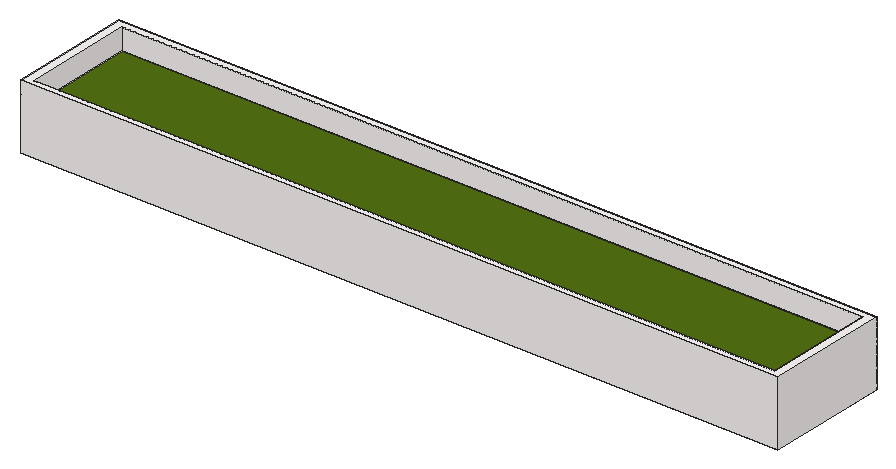
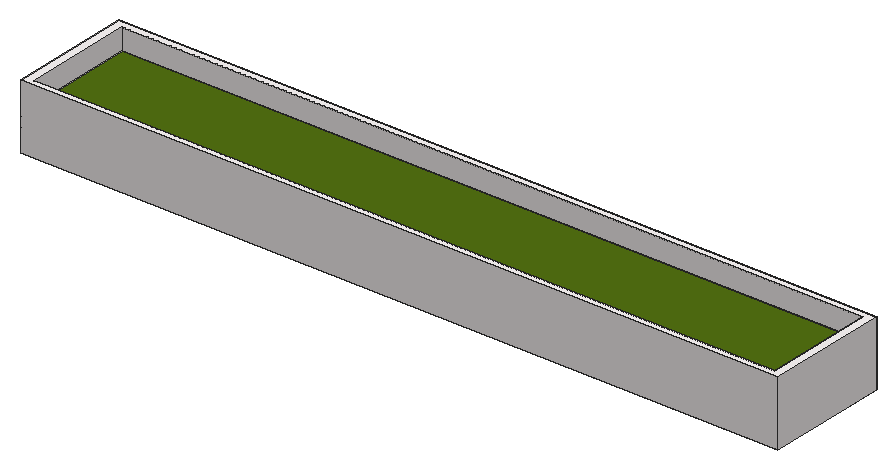
# SketchUp Ruby script. Lengths in inches.
U = 1.inch
M = Sketchup.active_model
def pt(a) = Geom::Point3d.new(a.map { |v| v * U })
def face(e, loops, mat)
  f = e.add_face(loops[0].map { |a| pt(a) })
  loops[1..].each { |l| e.add_face(l.map { |a| pt(a) }).erase! }
  f.material = f.back_material = mat if mat
  f
end
# faces: each face lists its corners as indices into pts; further lists are holes
def faces(e, pts, list, mat = nil) = list.each { |f| face(e, (f[0].is_a?(Array) ? f : [f]).map { |l| l.map { |i| pts[i] } }, mat) }
# xy, xz, yz: faces in a plane at the given z, y or x. An outline is a flat list of corners, or four numbers for a rectangle; further outlines are holes
def ring(l) = l.size == 4 ? [[l[0], l[1]], [l[2], l[1]], [l[2], l[3]], [l[0], l[3]]] : l.each_slice(2).to_a
def flat(e, list, mat, &to3) = list.each { |f| face(e, (f[0].is_a?(Array) ? f : [f]).map { |l| ring(l).map { |u, v| to3.(u, v) } }, mat) }
def xy(e, z, list, mat = nil) = flat(e, list, mat) { |x, y| [x, y, z] }
def xz(e, y, list, mat = nil) = flat(e, list, mat) { |x, z| [x, y, z] }
def yz(e, x, list, mat = nil) = flat(e, list, mat) { |y, z| [x, y, z] }
def lines(e, pts, list) = list.each { |a, b| e.add_line(pt(pts[a]), pt(pts[b])) }
# prism: a flat outline (further loops are holes) pulled along v
def prism(e, loops, v, mat = nil)
  f = face(e, loops, mat); d = Geom::Vector3d.new(v.map { |x| x * U })
  f.pushpull(f.normal.samedirection?(d) ? d.length : -d.length)
end
def box(e, o, s, mat = nil) = prism(e, [[o, [o[0] + s[0], o[1], o[2]], [o[0] + s[0], o[1] + s[1], o[2]], [o[0], o[1] + s[1], o[2]]]], [0, 0, s[2]], mat)
def at(x, y, z, deg = 0) = Geom::Transformation.translation(pt([x, y, z])) * Geom::Transformation.rotation(ORIGIN, Z_AXIS, deg.degrees)
def axes(o, x, y, z) = Geom::Transformation.new([*x, 0, *y, 0, *z, 0, *pt(o).to_a, 1])
def part(name) = M.definitions.add(name)
# library, detail: a bought-in or finely detailed component or shape, given as its bounding box
def library(name, o, s) = part(name).tap { |d| box(d.entities, o, s) }
def detail(e, o, s) = box(e.add_group.entities, o, s)
def put(e, d, t, mat = nil) = e.add_instance(d, t).tap { |i| i.material = mat if mat }
def group(e, t, mat = nil) = e.add_group.tap { |g| g.transformation = t; g.material = mat if mat }.entities
root = M.entities
M.materials.add("[0010_Snow]").color = [255, 250, 250]
M.materials.add("[Vegetation_Blur7]").color = [83, 114, 18]
xy(root,96.12,[[213.37,375.59,372.17,399.19]])
xy(root,96.12,[[[211.5,374.19,374.04,400.6],[213.37,375.59,372.17,399.19]]],"[0010_Snow]")
xy(root,105.39,[[213.37,375.59,372.17,399.19]],"[Vegetation_Blur7]")
xy(root,110.03,[[[211.5,374.19,374.04,400.6],[213.37,375.59,372.17,399.19]]],"[0010_Snow]")
xz(root,374.19,[[211.5,96.12,374.04,110.03]],"[0010_Snow]")
xz(root,375.59,[[213.37,96.12,372.17,105.39],[213.37,105.39,372.17,110.03]],"[0010_Snow]")
xz(root,399.19,[[213.37,96.12,372.17,105.39],[213.37,105.39,372.17,110.03]],"[0010_Snow]")
xz(root,400.6,[[211.5,96.12,374.04,110.03]],"[0010_Snow]")
yz(root,211.5,[[374.19,96.12,400.6,110.03]],"[0010_Snow]")
yz(root,213.37,[[375.59,96.12,399.19,105.39],[375.59,105.39,399.19,110.03]],"[0010_Snow]")
yz(root,372.17,[[375.59,96.12,399.19,105.39],[375.59,105.39,399.19,110.03]],"[0010_Snow]")
yz(root,374.04,[[374.19,96.12,400.6,110.03]],"[0010_Snow]")
